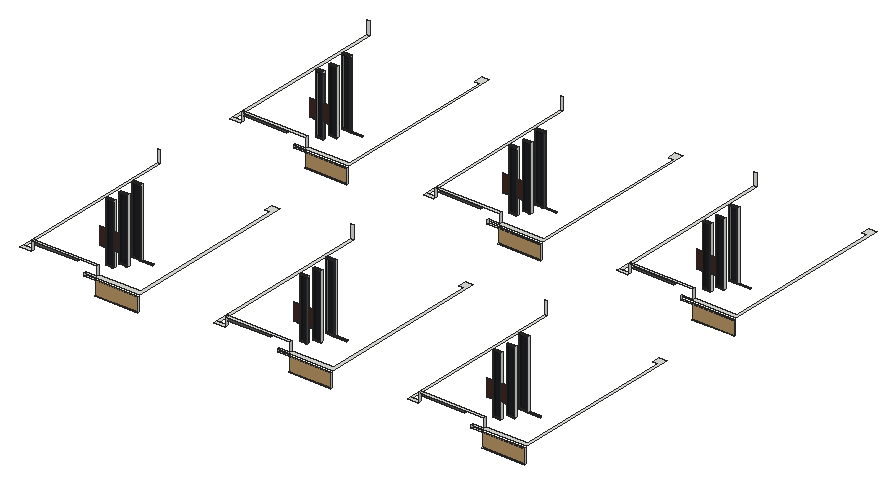
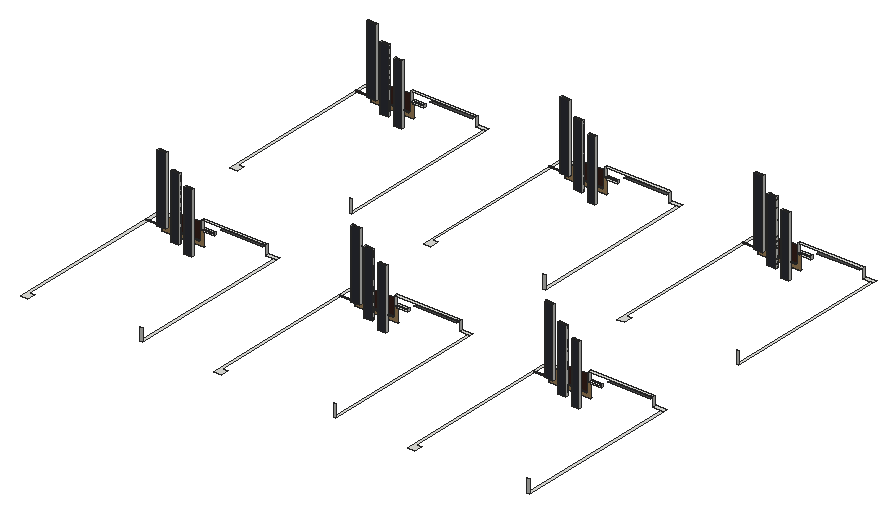
# SketchUp Ruby script. Lengths in inches.
U = 1.inch
M = Sketchup.active_model
def pt(a) = Geom::Point3d.new(a.map { |v| v * U })
def face(e, loops, mat)
  f = e.add_face(loops[0].map { |a| pt(a) })
  loops[1..].each { |l| e.add_face(l.map { |a| pt(a) }).erase! }
  f.material = f.back_material = mat if mat
  f
end
# faces: each face lists its corners as indices into pts; further lists are holes
def faces(e, pts, list, mat = nil) = list.each { |f| face(e, (f[0].is_a?(Array) ? f : [f]).map { |l| l.map { |i| pts[i] } }, mat) }
# xy, xz, yz: faces in a plane at the given z, y or x. An outline is a flat list of corners, or four numbers for a rectangle; further outlines are holes
def ring(l) = l.size == 4 ? [[l[0], l[1]], [l[2], l[1]], [l[2], l[3]], [l[0], l[3]]] : l.each_slice(2).to_a
def flat(e, list, mat, &to3) = list.each { |f| face(e, (f[0].is_a?(Array) ? f : [f]).map { |l| ring(l).map { |u, v| to3.(u, v) } }, mat) }
def xy(e, z, list, mat = nil) = flat(e, list, mat) { |x, y| [x, y, z] }
def xz(e, y, list, mat = nil) = flat(e, list, mat) { |x, z| [x, y, z] }
def yz(e, x, list, mat = nil) = flat(e, list, mat) { |y, z| [x, y, z] }
def lines(e, pts, list) = list.each { |a, b| e.add_line(pt(pts[a]), pt(pts[b])) }
# prism: a flat outline (further loops are holes) pulled along v
def prism(e, loops, v, mat = nil)
  f = face(e, loops, mat); d = Geom::Vector3d.new(v.map { |x| x * U })
  f.pushpull(f.normal.samedirection?(d) ? d.length : -d.length)
end
def box(e, o, s, mat = nil) = prism(e, [[o, [o[0] + s[0], o[1], o[2]], [o[0] + s[0], o[1] + s[1], o[2]], [o[0], o[1] + s[1], o[2]]]], [0, 0, s[2]], mat)
def at(x, y, z, deg = 0) = Geom::Transformation.translation(pt([x, y, z])) * Geom::Transformation.rotation(ORIGIN, Z_AXIS, deg.degrees)
def axes(o, x, y, z) = Geom::Transformation.new([*x, 0, *y, 0, *z, 0, *pt(o).to_a, 1])
def part(name) = M.definitions.add(name)
# library, detail: a bought-in or finely detailed component or shape, given as its bounding box
def library(name, o, s) = part(name).tap { |d| box(d.entities, o, s) }
def detail(e, o, s) = box(e.add_group.entities, o, s)
def put(e, d, t, mat = nil) = e.add_instance(d, t).tap { |i| i.material = mat if mat }
def group(e, t, mat = nil) = e.add_group.tap { |g| g.transformation = t; g.material = mat if mat }.entities
root = M.entities
M.materials.add("Glass_Tinted_Gray").color = [0, 0, 0]
M.materials["Glass_Tinted_Gray"].alpha = 0.125
M.materials.add("[0043_SaddleBrown]").color = [63, 38, 31]
M.materials.add("[0135_DarkGray]").color = [81, 81, 81]
M.materials.add("[Formica Laminate Dark]").color = [50, 53, 60]
M.materials.add("[Groundcover Sand Smooth]").color = [181, 147, 100]
M.materials.add("[Terrazzo Light Blue]").color = [196, 214, 227]
c1 = part("PENTEK_RP Fineline 50S_SlidingDoor_GlazingBead_2")
box(c1.entities,[0,0,0],[0.56,0.59,94.39],"[0135_DarkGray]")
c2 = part("PENTEK_RP Fineline 50S_SlidingDoor_Glass")
box(c2.entities,[0,0,0],[46.58,0.16,94.39],"Glass_Tinted_Gray")
c3 = part("PENTEK_RP Fineline 50S_SlidingDoor_GlazingBead")
box(c3.entities,[0,0,0],[45.47,0.59,0.56],"[0135_DarkGray]")
c4 = part("PENTEK_RP Fineline 50S_SlidingDoor_Leaf_E1")
xy(c4.entities,0,[[0,0,0.93,1.97],[0.93,1.57,1.49,1.97]],"[0135_DarkGray]")
xy(c4.entities,96.25,[[0,0,0.93,0,0.93,1.57,1.49,1.57,1.49,1.97,0,1.97]],"[0135_DarkGray]")
xz(c4.entities,0,[[0,0,0.93,96.25]],"[0135_DarkGray]")
xz(c4.entities,1.57,[[0.93,0,1.49,95.32],[0.93,95.32,1.49,96.25]],"[0135_DarkGray]")
xz(c4.entities,1.97,[[0,0,1.49,96.25]],"[0135_DarkGray]")
yz(c4.entities,0,[[0,0,1.97,96.25]],"[0135_DarkGray]")
yz(c4.entities,0.93,[[0,0,1.57,0.93],[0,0.93,1.57,95.32],[0,95.32,1.57,96.25]],"[0135_DarkGray]")
yz(c4.entities,1.49,[[1.57,0,1.97,95.32],[1.57,95.32,1.97,96.25]],"[0135_DarkGray]")
c5 = part("PENTEK_RP Fineline 50S_SlidingDoor_Leaf_E2")
xy(c5.entities,0,[[0,0,0,1.57,0.56,1.57,0.56,1.97,46.02,1.97,46.02,1.57,46.58,1.57,46.58,0]],"[0135_DarkGray]")
xy(c5.entities,0.93,[[0,0,46.58,1.57]],"[0135_DarkGray]")
xy(c5.entities,1.49,[[0.56,1.57,46.02,1.97]],"[0135_DarkGray]")
xz(c5.entities,0,[[0,0,46.58,0.93]],"[0135_DarkGray]")
xz(c5.entities,1.57,[[0,0,0.56,0.93],[46.02,0,46.58,0.93],[0.56,0.93,46.02,1.49]],"[0135_DarkGray]")
xz(c5.entities,1.97,[[0.56,0,46.02,1.49]],"[0135_DarkGray]")
yz(c5.entities,0,[[0,0,1.57,0.93]],"[0135_DarkGray]")
yz(c5.entities,0.56,[[1.57,0,1.97,0.93],[1.57,0.93,1.97,1.49]],"[0135_DarkGray]")
yz(c5.entities,46.02,[[1.57,0,1.97,0.93],[1.57,0.93,1.97,1.49]],"[0135_DarkGray]")
yz(c5.entities,46.58,[[0,0,1.57,0.93]],"[0135_DarkGray]")
c6 = part("PENTEK_RP Fineline S_SlidingDoor_Leaf1")
put(c6.entities,c1,at(0.93,0,0.93))
put(c6.entities,c1,at(46.96,0,0.93))
put(c6.entities,c2,at(1.49,1.42,0.93))
put(c6.entities,c3,at(1.49,0,0.93))
put(c6.entities,c2,at(1.49,0.59,0.93),"[Terrazzo Light Blue]")
put(c6.entities,c4,at(0,0,0))
put(c6.entities,c4,axes([48.44,0,0],[-1,0,0],[0,1,0],[0,0,1]))
put(c6.entities,c5,axes([0.93,0,96.25],[1,0,0],[0,1,0],[0,0,-1]))
put(c6.entities,c5,at(0.93,0,0))
put(c6.entities,c3,at(1.49,0,94.77))
xy(root,14.13,[[420.26,324.35,580.26,328.54],[1144.69,324.35,1304.69,328.54],[1869.13,324.35,2029.13,328.54],[420.26,1304.7,580.26,1308.89],[1144.69,1304.7,1304.69,1308.89],
  [1869.13,1304.7,2029.13,1308.89]])
xy(root,50.14,[[370.54,438.72,399.16,447.84],[1094.98,438.72,1123.6,447.84],[1819.41,438.72,1848.04,447.84],[370.54,1419.07,399.16,1428.19],[1094.98,1419.07,1123.6,1428.19],
  [1819.41,1419.07,1848.04,1428.19]])
xy(root,67.07,[[379.07,324.35,420.26,332.35],[420.26,324.35,580.26,328.54],[1103.51,324.35,1144.69,332.35],[1144.69,324.35,1304.69,328.54],[1827.94,324.35,1869.13,332.35],
  [1869.13,324.35,2029.13,328.54],[379.07,1304.7,420.26,1312.7],[420.26,1304.7,580.26,1308.89],[1103.51,1304.7,1144.69,1312.7],[1144.69,1304.7,1304.69,1308.89],
  [1827.94,1304.7,1869.13,1312.7],[1869.13,1304.7,2029.13,1308.89]])
xy(root,73.83,[[419.76,438.72,451.01,447.84],[1144.2,438.72,1175.45,447.84],[1868.64,438.72,1899.89,447.84],[419.76,1419.07,451.01,1428.19],[1144.2,1419.07,1175.45,1428.19],
  [1868.64,1419.07,1899.89,1428.19]])
xy(root,77.97,[[379.07,324.35,586.9375,324.35,586.9375,980.35,558.625,980.35,558.625,948.22,577.26,948.22,577.26,341.79,420.26,341.79,420.26,332.35,379.07,332.35],[1103.51,324.35,1311.375,324.35,1311.375,980.35,1283.0625,980.35,1283.0625,948.22,1301.69,948.22,1301.69,341.79,1144.69,341.79,1144.69,332.35,1103.51,332.35],[1827.94,324.35,2035.8125,324.35,2035.8125,980.35,2007.5,980.35,2007.5,948.22,2026.13,948.22,2026.13,341.79,1869.13,341.79,1869.13,332.35,1827.94,332.35],[137.5,328.54,177.74,343.16],[861.9375,328.54,902.18,343.16],
  [1586.375,328.54,1626.62,343.16],[137.5,343.16,146.62,971.23],[861.9375,343.16,871.06,971.23],[1586.375,343.16,1595.49,971.23],[379.07,1304.7,586.9375,1304.7,586.9375,1960.7,558.625,1960.7,558.625,1928.57,577.26,1928.57,577.26,1322.14,420.26,1322.14,420.26,1312.7,379.07,1312.7],
  [1103.51,1304.7,1311.375,1304.7,1311.375,1960.7,1283.0625,1960.7,1283.0625,1928.57,1301.69,1928.57,1301.69,1322.14,1144.69,1322.14,1144.69,1312.7,1103.51,1312.7],[1827.94,1304.7,2035.8125,1304.7,2035.8125,1960.7,2007.5,1960.7,2007.5,1928.57,2026.13,1928.57,2026.13,1322.14,1869.13,1322.14,1869.13,1312.7,1827.94,1312.7],[137.5,1308.89,177.74,1323.51],[861.9375,1308.89,902.18,1323.51],[1586.375,1308.89,1626.62,1323.51],
  [137.5,1323.51,146.62,1951.58],[861.9375,1323.51,871.06,1951.58],[1586.375,1323.51,1595.49,1951.58]])
xy(root,102.02,[[188.43,332.35,348.44,341.79],[912.87,332.35,1072.88,341.79],[1637.31,332.35,1797.32,341.79],[188.43,1312.7,348.44,1322.14],[912.87,1312.7,1072.88,1322.14],
  [1637.31,1312.7,1797.32,1322.14]],"[0135_DarkGray]")
xy(root,109.76,[[348.1875,438.72,370.54,441.04],[1072.625,438.72,1094.98,441.04],[1797.0625,438.72,1819.41,441.04],[348.1875,1419.07,370.54,1419.08,370.54,1421.39,348.1875,1421.39],[1072.625,1419.07,1094.98,1419.08,1094.98,1421.39,1072.625,1421.39],
  [1797.0625,1419.07,1819.41,1419.08,1819.41,1421.39,1797.0625,1421.39]])
xy(root,109.99,[[419.76,438.72,419.76,441.04,399.16,441.04,399.16,438.73],[1144.2,438.72,1144.2,441.04,1123.6,441.04,1123.6,438.73],[1868.64,438.72,1868.64,441.04,1848.04,441.04,1848.04,438.73],[419.76,1419.07,419.76,1421.39,399.16,1421.39,399.16,1419.08],[1144.2,1419.07,1144.2,1421.39,1123.6,1421.39,1123.6,1419.08],
  [1868.64,1419.07,1868.64,1421.39,1848.04,1421.39,1848.04,1419.08]])
xy(root,110.73,[[467.3,438.72,500.42,447.84],[500.42,438.72,547.05,441.04],[1191.74,438.72,1224.86,447.84],[1224.86,438.72,1271.49,441.04],[1916.17,438.72,1949.3,447.84],
  [1949.3,438.72,1995.93,441.04],[467.3,1419.07,500.42,1428.19],[500.42,1419.07,547.05,1421.39],[1191.74,1419.07,1224.86,1428.19],[1224.86,1419.07,1271.49,1421.39],
  [1916.17,1419.07,1949.3,1428.19],[1949.3,1419.07,1995.93,1421.39]])
xy(root,111.97,[[177.74,332.35,188.43,341.79],[188.43,332.35,420.26,341.79],[902.18,332.35,912.87,341.79],[912.87,332.35,1144.69,341.79],[1626.62,332.35,1637.31,341.79],
  [1637.31,332.35,1869.13,341.79],[177.74,1312.7,188.43,1322.14],[188.43,1312.7,420.26,1322.14],[902.18,1312.7,912.87,1322.14],[912.87,1312.7,1144.69,1322.14],
  [1626.62,1312.7,1637.31,1322.14],[1637.31,1312.7,1869.13,1322.14]])
xy(root,112.41,[[348.1875,438.72,370.54,441.04],[1072.625,438.72,1094.98,441.04],[1797.0625,438.72,1819.41,441.04],[348.1875,1419.07,370.54,1421.39],[1072.625,1419.07,1094.98,1421.39],
  [1797.0625,1419.07,1819.41,1421.39]])
xy(root,113.69,[[419.76,438.72,399.16,438.73,399.16,441.04,419.76,441.04],[1144.2,438.72,1123.6,438.73,1123.6,441.04,1144.2,441.04],[1868.64,438.72,1848.04,438.73,1848.04,441.04,1868.64,441.04],[419.76,1419.07,399.16,1419.08,399.16,1421.39,419.76,1421.39],[1144.2,1419.07,1123.6,1419.08,1123.6,1421.39,1144.2,1421.39],
  [1868.64,1419.07,1848.04,1419.08,1848.04,1421.39,1868.64,1421.39]])
xz(root,328.54,[[420.26,14.13,580.26,67.07],[1144.69,14.13,1304.69,67.07],[1869.13,14.13,2029.13,67.07]],"[Groundcover Sand Smooth]")
xz(root,438.72,[[348.1875,112.41,370.54,174.69],[1072.625,112.41,1094.98,174.69],[1797.0625,112.41,1819.41,174.69]],"[0043_SaddleBrown]")
xz(root,441.04,[[348.1875,109.76,370.54,112.41],[1072.625,109.76,1094.98,112.41],[1797.0625,109.76,1819.41,112.41],[399.16,109.99,419.76,113.69],[1123.6,109.99,1144.2,113.69],
  [1848.04,109.99,1868.64,113.69],[500.42,110.73,547.05,114.29],[1224.86,110.73,1271.49,114.29],[1949.3,110.73,1995.93,114.29]],"[0043_SaddleBrown]")
xz(root,447.84,[[370.54,50.14,399.16,275.89],[1094.98,50.14,1123.6,275.89],[1819.41,50.14,1848.04,275.89],[419.76,73.83,451.01,312.4],[1144.2,73.83,1175.45,312.4],
  [1868.64,73.83,1899.89,312.4],[467.3,110.73,500.42,365.23],[1191.74,110.73,1224.86,365.23],[1916.17,110.73,1949.3,365.23]],"[Formica Laminate Dark]")
xz(root,971.23,[[137.5,77.97,146.62,126.125],[861.9375,77.97,871.06,126.125],[1586.375,77.97,1595.49,126.125]])
xz(root,1308.89,[[420.26,14.13,580.26,67.07],[1144.69,14.13,1304.69,67.07],[1869.13,14.13,2029.13,67.07]],"[Groundcover Sand Smooth]")
xz(root,1421.39,[[348.1875,109.76,370.54,112.41],[1072.625,109.76,1094.98,112.41],[1797.0625,109.76,1819.41,112.41],[399.16,109.99,419.76,113.69],[1123.6,109.99,1144.2,113.69],
  [1848.04,109.99,1868.64,113.69],[500.42,110.73,547.05,114.29],[1224.86,110.73,1271.49,114.29],[1949.3,110.73,1995.93,114.29]],"[0043_SaddleBrown]")
xz(root,1428.19,[[370.54,50.14,399.16,275.89],[1094.98,50.14,1123.6,275.89],[1819.41,50.14,1848.04,275.89],[419.76,73.83,451.01,312.4],[1144.2,73.83,1175.45,312.4],
  [1868.64,73.83,1899.89,312.4],[467.3,110.73,500.42,365.23],[1191.74,110.73,1224.86,365.23],[1916.17,110.73,1949.3,365.23]],"[Formica Laminate Dark]")
xz(root,1951.58,[[137.5,77.97,146.62,126.125],[861.9375,77.97,871.06,126.125],[1586.375,77.97,1595.49,126.125]])
yz(root,177.74,[[332.35,77.97,341.79,111.97],[1312.7,77.97,1322.14,111.97]])
yz(root,370.54,[[438.72,50.14,447.84,50.14,447.84,275.89,438.72,275.89,438.72,246.4375,441.04,246.4375,441.04,243.96,438.72,243.96,438.72,176.39,441.04,176.39,441.04,174.69,438.72,174.69,438.72,112.41,441.04,112.41,441.04,109.76,438.72,109.76],[1419.07,50.14,1428.19,50.14,1428.19,275.89,1419.07,275.89,1419.07,246.4375,1421.39,246.4375,1421.39,243.96,1419.07,243.96,1419.07,176.39,1421.39,176.39,1421.39,174.69,1419.08,174.69,1419.07,112.41,1421.39,112.41,1421.39,109.76,1419.08,109.76]])
yz(root,379.07,[[324.35,67.07,332.35,77.97],[1304.7,67.07,1312.7,77.97]])
yz(root,399.16,[[438.72,50.14,438.73,109.99,441.04,109.99,441.04,113.69,438.73,113.69,438.73,173.87,441.04,173.87,441.04,175.12,438.73,175.12,438.72,243.96,441.04,243.96,441.04,246.18,438.72,246.18,438.72,275.89,447.84,275.89,447.84,50.14],[1419.07,50.14,1419.08,109.99,1421.39,109.99,1421.39,113.69,1419.08,113.69,1419.08,173.87,1421.39,173.87,1421.39,175.12,1419.08,175.12,1419.07,243.96,1421.39,243.96,1421.39,246.18,1419.07,246.18,1419.07,275.89,1428.19,275.89,1428.19,50.14]])
yz(root,419.76,[[438.72,73.83,447.84,73.83,447.84,312.4,438.72,312.4,438.72,306.15,441.04,306.15,441.04,303,438.72,303,438.72,246.18,441.04,246.18,441.04,243.96,438.72,243.96,438.72,175.12,441.04,175.12,441.04,173.87,438.72,173.87,438.72,113.69,441.04,113.69,441.04,109.99,438.72,109.99],[1419.07,73.83,1428.19,73.83,1428.19,312.4,1419.07,312.4,1419.08,306.15,1421.39,306.15,1421.39,303,1419.07,303,1419.07,246.18,1421.39,246.18,1421.39,243.96,1419.07,243.96,1419.07,175.12,1421.39,175.12,1421.39,173.87,1419.07,173.87,1419.07,113.69,1421.39,113.69,1421.39,109.99,1419.07,109.99]])
yz(root,420.26,[[332.35,77.97,341.79,111.97],[1312.7,77.97,1322.14,111.97]])
yz(root,451.01,[[438.72,73.83,438.72,173.82,441.04,173.82,441.04,175.93,438.72,175.93,438.72,243.96,441.04,243.96,441.04,245.59,438.72,245.59,438.72,303,441.04,303,441.04,306.93,438.72,306.93,438.72,312.4,447.84,312.4,447.84,73.83],[1419.07,73.83,1419.07,173.82,1421.39,173.82,1421.39,175.93,1419.07,175.93,1419.07,243.96,1421.39,243.96,1421.39,245.59,1419.07,245.59,1419.07,303,1421.39,303,1421.39,306.93,1419.07,306.93,1419.07,312.4,1428.19,312.4,1428.19,73.83]])
yz(root,467.3,[[438.72,110.73,447.84,110.73,447.84,365.23,438.72,365.23,438.72,355.72,441.04,355.72,441.04,354.05,438.72,354.05,438.72,306.93,441.04,306.93,441.04,303,438.72,303,438.72,245.59,441.04,245.59,441.04,243.96,438.72,243.96,438.72,175.93,441.04,175.93,441.04,173.82,438.72,173.82],[1419.07,110.73,1428.19,110.73,1428.19,365.23,1419.07,365.23,1419.07,355.72,1421.39,355.72,1421.39,354.05,1419.07,354.05,1419.07,306.93,1421.39,306.93,1421.39,303,1419.07,303,1419.07,245.59,1421.39,245.59,1421.39,243.96,1419.07,243.96,1419.07,175.93,1421.39,175.93,1421.39,173.82,1419.07,173.82]])
yz(root,500.42,[[441.04,110.73,441.04,114.29,438.72,114.29,438.73,174.81,441.04,174.81,441.04,177.22,438.73,177.22,438.73,243.96,441.04,243.96,441.04,246.28,438.73,246.28,438.73,303,441.04,303,441.04,306.7,438.73,306.7,438.73,354.27,441.04,354.27,441.04,357.3,438.73,357.3,438.72,365.23,447.84,365.23,447.84,110.73],[1421.39,110.73,1421.39,114.29,1419.07,114.29,1419.08,174.81,1421.39,174.81,1421.39,177.22,1419.08,177.22,1419.08,243.96,1421.39,243.96,1421.39,246.28,1419.08,246.28,1419.08,303,1421.39,303,1421.39,306.7,1419.08,306.7,1419.08,354.27,1421.39,354.27,1421.39,357.3,1419.08,357.3,1419.07,365.23,1428.19,365.23,1428.19,110.73]])
yz(root,580.26,[[324.35,14.13,328.54,67.07],[1304.7,14.13,1308.89,67.07]])
yz(root,902.18,[[332.35,77.97,341.79,111.97],[1312.7,77.97,1322.14,111.97]])
yz(root,1094.98,[[438.72,50.14,447.84,50.14,447.84,275.89,438.72,275.89,438.72,246.4375,441.04,246.4375,441.04,243.96,438.72,243.96,438.72,176.39,441.04,176.39,441.04,174.69,438.72,174.69,438.72,112.41,441.04,112.41,441.04,109.76,438.72,109.76],[1419.07,50.14,1428.19,50.14,1428.19,275.89,1419.07,275.89,1419.07,246.4375,1421.39,246.4375,1421.39,243.96,1419.07,243.96,1419.07,176.39,1421.39,176.39,1421.39,174.69,1419.08,174.69,1419.07,112.41,1421.39,112.41,1421.39,109.76,1419.08,109.76]])
yz(root,1103.51,[[324.35,67.07,332.35,77.97],[1304.7,67.07,1312.7,77.97]])
yz(root,1123.6,[[438.72,50.14,438.73,109.99,441.04,109.99,441.04,113.69,438.73,113.69,438.73,173.87,441.04,173.87,441.04,175.12,438.73,175.12,438.72,243.96,441.04,243.96,441.04,246.18,438.72,246.18,438.72,275.89,447.84,275.89,447.84,50.14],[1419.07,50.14,1419.08,109.99,1421.39,109.99,1421.39,113.69,1419.08,113.69,1419.08,173.87,1421.39,173.87,1421.39,175.12,1419.08,175.12,1419.07,243.96,1421.39,243.96,1421.39,246.18,1419.07,246.18,1419.07,275.89,1428.19,275.89,1428.19,50.14]])
yz(root,1144.2,[[438.72,73.83,447.84,73.83,447.84,312.4,438.72,312.4,438.72,306.15,441.04,306.15,441.04,303,438.72,303,438.72,246.18,441.04,246.18,441.04,243.96,438.72,243.96,438.72,175.12,441.04,175.12,441.04,173.87,438.72,173.87,438.72,113.69,441.04,113.69,441.04,109.99,438.72,109.99],[1419.07,73.83,1428.19,73.83,1428.19,312.4,1419.07,312.4,1419.08,306.15,1421.39,306.15,1421.39,303,1419.07,303,1419.07,246.18,1421.39,246.18,1421.39,243.96,1419.07,243.96,1419.07,175.12,1421.39,175.12,1421.39,173.87,1419.07,173.87,1419.07,113.69,1421.39,113.69,1421.39,109.99,1419.07,109.99]])
yz(root,1144.69,[[332.35,77.97,341.79,111.97],[1312.7,77.97,1322.14,111.97]])
yz(root,1175.45,[[438.72,73.83,438.72,173.82,441.04,173.82,441.04,175.93,438.72,175.93,438.72,243.96,441.04,243.96,441.04,245.59,438.72,245.59,438.72,303,441.04,303,441.04,306.93,438.72,306.93,438.72,312.4,447.84,312.4,447.84,73.83],[1419.07,73.83,1419.07,173.82,1421.39,173.82,1421.39,175.93,1419.07,175.93,1419.07,243.96,1421.39,243.96,1421.39,245.59,1419.07,245.59,1419.07,303,1421.39,303,1421.39,306.93,1419.07,306.93,1419.07,312.4,1428.19,312.4,1428.19,73.83]])
yz(root,1191.74,[[438.72,110.73,447.84,110.73,447.84,365.23,438.72,365.23,438.72,355.72,441.04,355.72,441.04,354.05,438.72,354.05,438.72,306.93,441.04,306.93,441.04,303,438.72,303,438.72,245.59,441.04,245.59,441.04,243.96,438.72,243.96,438.72,175.93,441.04,175.93,441.04,173.82,438.72,173.82],[1419.07,110.73,1428.19,110.73,1428.19,365.23,1419.07,365.23,1419.07,355.72,1421.39,355.72,1421.39,354.05,1419.07,354.05,1419.07,306.93,1421.39,306.93,1421.39,303,1419.07,303,1419.07,245.59,1421.39,245.59,1421.39,243.96,1419.07,243.96,1419.07,175.93,1421.39,175.93,1421.39,173.82,1419.07,173.82]])
yz(root,1224.86,[[441.04,110.73,441.04,114.29,438.72,114.29,438.73,174.81,441.04,174.81,441.04,177.22,438.73,177.22,438.73,243.96,441.04,243.96,441.04,246.28,438.73,246.28,438.73,303,441.04,303,441.04,306.7,438.73,306.7,438.73,354.27,441.04,354.27,441.04,357.3,438.73,357.3,438.72,365.23,447.84,365.23,447.84,110.73],[1421.39,110.73,1421.39,114.29,1419.07,114.29,1419.08,174.81,1421.39,174.81,1421.39,177.22,1419.08,177.22,1419.08,243.96,1421.39,243.96,1421.39,246.28,1419.08,246.28,1419.08,303,1421.39,303,1421.39,306.7,1419.08,306.7,1419.08,354.27,1421.39,354.27,1421.39,357.3,1419.08,357.3,1419.07,365.23,1428.19,365.23,1428.19,110.73]])
yz(root,1304.69,[[324.35,14.13,328.54,67.07],[1304.7,14.13,1308.89,67.07]])
yz(root,1626.62,[[332.35,77.97,341.79,111.97],[1312.7,77.97,1322.14,111.97]])
yz(root,1819.41,[[438.72,50.14,447.84,50.14,447.84,275.89,438.72,275.89,438.72,246.4375,441.04,246.4375,441.04,243.96,438.72,243.96,438.72,176.39,441.04,176.39,441.04,174.69,438.72,174.69,438.72,112.41,441.04,112.41,441.04,109.76,438.72,109.76],[1419.07,50.14,1428.19,50.14,1428.19,275.89,1419.07,275.89,1419.07,246.4375,1421.39,246.4375,1421.39,243.96,1419.07,243.96,1419.07,176.39,1421.39,176.39,1421.39,174.69,1419.08,174.69,1419.07,112.41,1421.39,112.41,1421.39,109.76,1419.08,109.76]])
yz(root,1827.94,[[324.35,67.07,332.35,77.97],[1304.7,67.07,1312.7,77.97]])
yz(root,1848.04,[[438.72,50.14,438.73,109.99,441.04,109.99,441.04,113.69,438.73,113.69,438.73,173.87,441.04,173.87,441.04,175.12,438.73,175.12,438.72,243.96,441.04,243.96,441.04,246.18,438.72,246.18,438.72,275.89,447.84,275.89,447.84,50.14],[1419.07,50.14,1419.08,109.99,1421.39,109.99,1421.39,113.69,1419.08,113.69,1419.08,173.87,1421.39,173.87,1421.39,175.12,1419.08,175.12,1419.07,243.96,1421.39,243.96,1421.39,246.18,1419.07,246.18,1419.07,275.89,1428.19,275.89,1428.19,50.14]])
yz(root,1868.64,[[438.72,73.83,447.84,73.83,447.84,312.4,438.72,312.4,438.72,306.15,441.04,306.15,441.04,303,438.72,303,438.72,246.18,441.04,246.18,441.04,243.96,438.72,243.96,438.72,175.12,441.04,175.12,441.04,173.87,438.72,173.87,438.72,113.69,441.04,113.69,441.04,109.99,438.72,109.99],[1419.07,73.83,1428.19,73.83,1428.19,312.4,1419.07,312.4,1419.08,306.15,1421.39,306.15,1421.39,303,1419.07,303,1419.07,246.18,1421.39,246.18,1421.39,243.96,1419.07,243.96,1419.07,175.12,1421.39,175.12,1421.39,173.87,1419.07,173.87,1419.07,113.69,1421.39,113.69,1421.39,109.99,1419.07,109.99]])
yz(root,1869.13,[[332.35,77.97,341.79,111.97],[1312.7,77.97,1322.14,111.97]])
yz(root,1899.89,[[438.72,73.83,438.72,173.82,441.04,173.82,441.04,175.93,438.72,175.93,438.72,243.96,441.04,243.96,441.04,245.59,438.72,245.59,438.72,303,441.04,303,441.04,306.93,438.72,306.93,438.72,312.4,447.84,312.4,447.84,73.83],[1419.07,73.83,1419.07,173.82,1421.39,173.82,1421.39,175.93,1419.07,175.93,1419.07,243.96,1421.39,243.96,1421.39,245.59,1419.07,245.59,1419.07,303,1421.39,303,1421.39,306.93,1419.07,306.93,1419.07,312.4,1428.19,312.4,1428.19,73.83]])
yz(root,1916.17,[[438.72,110.73,447.84,110.73,447.84,365.23,438.72,365.23,438.72,355.72,441.04,355.72,441.04,354.05,438.72,354.05,438.72,306.93,441.04,306.93,441.04,303,438.72,303,438.72,245.59,441.04,245.59,441.04,243.96,438.72,243.96,438.72,175.93,441.04,175.93,441.04,173.82,438.72,173.82],[1419.07,110.73,1428.19,110.73,1428.19,365.23,1419.07,365.23,1419.07,355.72,1421.39,355.72,1421.39,354.05,1419.07,354.05,1419.07,306.93,1421.39,306.93,1421.39,303,1419.07,303,1419.07,245.59,1421.39,245.59,1421.39,243.96,1419.07,243.96,1419.07,175.93,1421.39,175.93,1421.39,173.82,1419.07,173.82]])
yz(root,1949.3,[[441.04,110.73,441.04,114.29,438.72,114.29,438.73,174.81,441.04,174.81,441.04,177.22,438.73,177.22,438.73,243.96,441.04,243.96,441.04,246.28,438.73,246.28,438.73,303,441.04,303,441.04,306.7,438.73,306.7,438.73,354.27,441.04,354.27,441.04,357.3,438.73,357.3,438.72,365.23,447.84,365.23,447.84,110.73],[1421.39,110.73,1421.39,114.29,1419.07,114.29,1419.08,174.81,1421.39,174.81,1421.39,177.22,1419.08,177.22,1419.08,243.96,1421.39,243.96,1421.39,246.28,1419.08,246.28,1419.08,303,1421.39,303,1421.39,306.7,1419.08,306.7,1419.08,354.27,1421.39,354.27,1421.39,357.3,1419.08,357.3,1419.07,365.23,1428.19,365.23,1428.19,110.73]])
yz(root,2029.13,[[324.35,14.13,328.54,67.07],[1304.7,14.13,1308.89,67.07]])
p = [[348.1875,1419.07,126.125],[348.1875,1419.07,112.41],[370.54,1419.07,112.41],[370.54,1419.08,174.69],[348.1875,1419.07,174.69],[348.1875,1419.07,143.875],
  [348.1875,1419.07,132.25],[1072.625,1419.07,126.125],[1072.625,1419.07,112.41],[1094.98,1419.07,112.41],[1094.98,1419.08,174.69],[1072.625,1419.07,174.69],
  [1072.625,1419.07,143.875],[1072.625,1419.07,132.25],[1797.0625,1419.07,126.125],[1797.0625,1419.07,112.41],[1819.41,1419.07,112.41],[1819.41,1419.08,174.69],
  [1797.0625,1419.07,174.69],[1797.0625,1419.07,143.875],[1797.0625,1419.07,132.25],[399.16,438.73,173.87],[399.16,438.73,113.69],[419.76,438.72,113.69],
  [419.76,438.72,173.87],[1123.6,438.73,173.87],[1123.6,438.73,113.69],[1144.2,438.72,113.69],[1144.2,438.72,173.87],[1848.04,438.73,173.87],
  [1848.04,438.73,113.69],[1868.64,438.72,113.69],[1868.64,438.72,173.87],[399.16,1419.08,173.87],[399.16,1419.08,113.69],[419.76,1419.07,113.69],
  [419.76,1419.07,173.87],[1123.6,1419.08,173.87],[1123.6,1419.08,113.69],[1144.2,1419.07,113.69],[1144.2,1419.07,173.87],[1848.04,1419.08,173.87],
  [1848.04,1419.08,113.69],[1868.64,1419.07,113.69],[1868.64,1419.07,173.87]]
faces(root,p,[[0,1,2,3,4,5,6],[7,8,9,10,11,12,13],[14,15,16,17,18,19,20],[21,22,23,24],[25,26,27,28],[29,30,31,32],[33,34,35,36],[37,38,39,40],
  [41,42,43,44]],"[0043_SaddleBrown]")
put(root,c6,axes([370.54,1419.07,50.14],[0.59088,0,0],[0,1,0],[0,0,2.34535]))
put(root,c6,axes([1094.98,1419.07,50.14],[0.59088,0,0],[0,1,0],[0,0,2.34535]))
put(root,c6,axes([1819.41,1419.07,50.14],[0.59088,0,0],[0,1,0],[0,0,2.34535]))
put(root,c6,axes([1094.98,438.72,50.14],[0.59088,0,0],[0,1,0],[0,0,2.34535]))
put(root,c6,axes([1819.41,438.72,50.14],[0.59088,0,0],[0,1,0],[0,0,2.34535]))
put(root,c6,axes([370.54,438.72,50.14],[0.59088,0,0],[0,1,0],[0,0,2.34535]))
put(root,c6,axes([419.76,1419.07,73.1],[0.64406,0,0],[0,1,0],[0,0,2.48607]))
put(root,c6,axes([1144.2,1419.07,73.1],[0.64406,0,0],[0,1,0],[0,0,2.48607]))
put(root,c6,axes([1868.64,1419.07,73.1],[0.64406,0,0],[0,1,0],[0,0,2.48607]))
put(root,c6,axes([1144.2,438.72,73.1],[0.64406,0,0],[0,1,0],[0,0,2.48607]))
put(root,c6,axes([1868.64,438.72,73.1],[0.64406,0,0],[0,1,0],[0,0,2.48607]))
put(root,c6,axes([419.76,438.72,73.1],[0.64406,0,0],[0,1,0],[0,0,2.48607]))
put(root,c6,axes([1191.74,1419.07,110.73],[0.68377,0,0],[0,1,0],[0,0,2.64403]))
put(root,c6,axes([1916.17,1419.07,110.73],[0.68377,0,0],[0,1,0],[0,0,2.64403]))
put(root,c6,axes([467.3,1419.07,110.73],[0.68377,0,0],[0,1,0],[0,0,2.64403]))
put(root,c6,axes([1191.74,438.72,110.73],[0.68377,0,0],[0,1,0],[0,0,2.64403]))
put(root,c6,axes([1916.17,438.72,110.73],[0.68377,0,0],[0,1,0],[0,0,2.64403]))
put(root,c6,axes([467.3,438.72,110.73],[0.68377,0,0],[0,1,0],[0,0,2.64403]))
